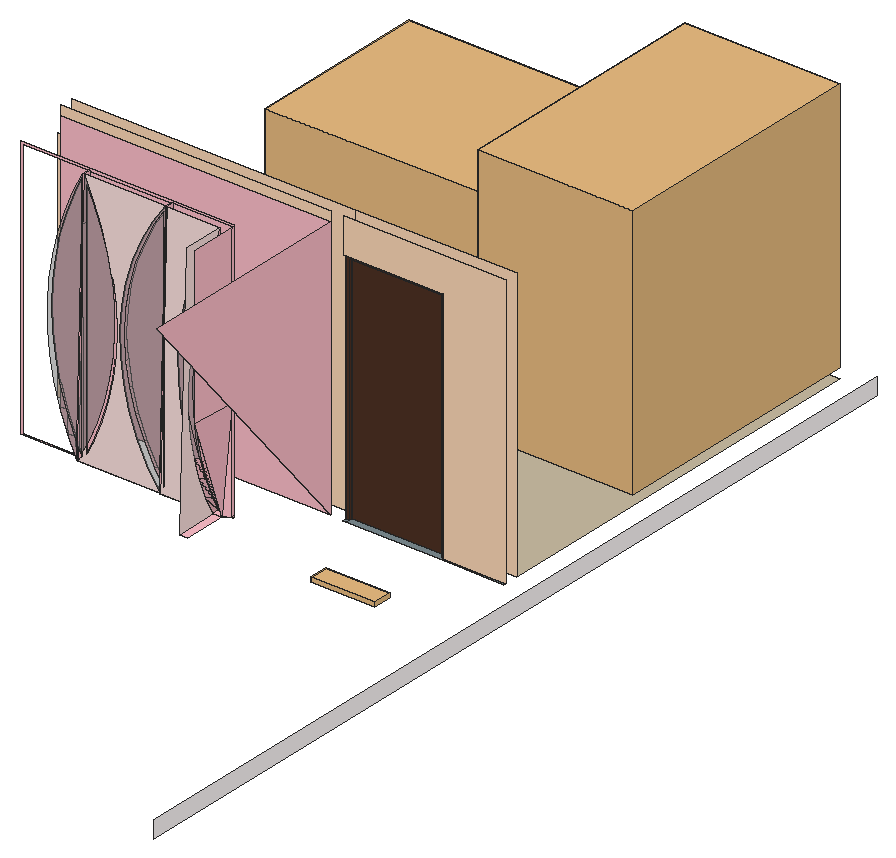
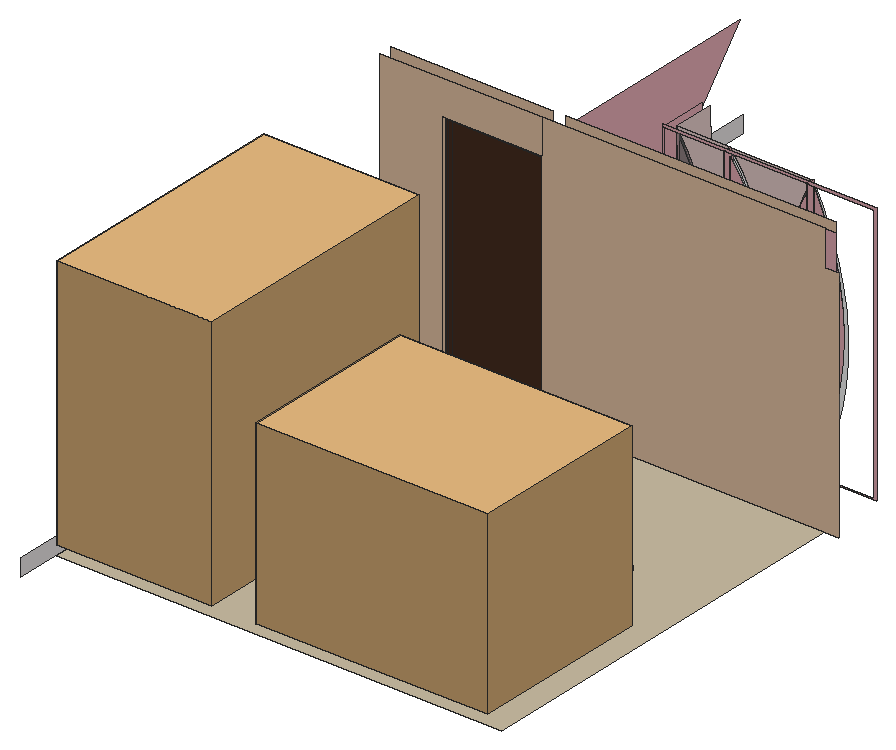
# SketchUp Ruby script. Lengths in inches.
U = 1.inch
M = Sketchup.active_model
def pt(a) = Geom::Point3d.new(a.map { |v| v * U })
def face(e, loops, mat)
  f = e.add_face(loops[0].map { |a| pt(a) })
  loops[1..].each { |l| e.add_face(l.map { |a| pt(a) }).erase! }
  f.material = f.back_material = mat if mat
  f
end
# faces: each face lists its corners as indices into pts; further lists are holes
def faces(e, pts, list, mat = nil) = list.each { |f| face(e, (f[0].is_a?(Array) ? f : [f]).map { |l| l.map { |i| pts[i] } }, mat) }
# xy, xz, yz: faces in a plane at the given z, y or x. An outline is a flat list of corners, or four numbers for a rectangle; further outlines are holes
def ring(l) = l.size == 4 ? [[l[0], l[1]], [l[2], l[1]], [l[2], l[3]], [l[0], l[3]]] : l.each_slice(2).to_a
def flat(e, list, mat, &to3) = list.each { |f| face(e, (f[0].is_a?(Array) ? f : [f]).map { |l| ring(l).map { |u, v| to3.(u, v) } }, mat) }
def xy(e, z, list, mat = nil) = flat(e, list, mat) { |x, y| [x, y, z] }
def xz(e, y, list, mat = nil) = flat(e, list, mat) { |x, z| [x, y, z] }
def yz(e, x, list, mat = nil) = flat(e, list, mat) { |y, z| [x, y, z] }
def lines(e, pts, list) = list.each { |a, b| e.add_line(pt(pts[a]), pt(pts[b])) }
# prism: a flat outline (further loops are holes) pulled along v
def prism(e, loops, v, mat = nil)
  f = face(e, loops, mat); d = Geom::Vector3d.new(v.map { |x| x * U })
  f.pushpull(f.normal.samedirection?(d) ? d.length : -d.length)
end
def box(e, o, s, mat = nil) = prism(e, [[o, [o[0] + s[0], o[1], o[2]], [o[0] + s[0], o[1] + s[1], o[2]], [o[0], o[1] + s[1], o[2]]]], [0, 0, s[2]], mat)
def at(x, y, z, deg = 0) = Geom::Transformation.translation(pt([x, y, z])) * Geom::Transformation.rotation(ORIGIN, Z_AXIS, deg.degrees)
def axes(o, x, y, z) = Geom::Transformation.new([*x, 0, *y, 0, *z, 0, *pt(o).to_a, 1])
def part(name) = M.definitions.add(name)
# library, detail: a bought-in or finely detailed component or shape, given as its bounding box
def library(name, o, s) = part(name).tap { |d| box(d.entities, o, s) }
def detail(e, o, s) = box(e.add_group.entities, o, s)
def put(e, d, t, mat = nil) = e.add_instance(d, t).tap { |i| i.material = mat if mat }
def group(e, t, mat = nil) = e.add_group.tap { |g| g.transformation = t; g.material = mat if mat }.entities
root = M.entities
M.materials.add("Polis06_194").color = [79, 50, 36]
M.materials.add("[0006_Pink]").color = [255, 192, 203]
M.materials.add("[0007_MistyRose]").color = [255, 228, 225]
M.materials.add("[0010_Snow]").color = [255, 250, 250]
M.materials.add("[0027_PeachPuff]").color = [255, 218, 185]
M.materials.add("[0093_AliceBlue]").color = [240, 248, 255]
M.materials.add("[Concrete Pavers Block Multi]").color = [124, 140, 145]
M.materials.add("[Concrete Tile]").color = [203, 190, 164]
M.materials.add("[Translucent Glass Gray]").color = [128, 128, 128]
M.materials["[Translucent Glass Gray]"].alpha = 0.5
c1 = library("Bedroom1",[0.98,0,0],[44.34,8.22,2])
c2 = library("Bed 003",[-38.05,-87.1,0],[75.86,87.1,55.12])
c3 = part("Flush door")
xy(c3.entities,0,[[0,0,4.72,1.18],[0,34.25,4.72,35.43]],"Polis06_194")
xy(c3.entities,85.26,[[0,1.18,4.72,34.25]],"Polis06_194")
xy(c3.entities,86.61,[[0,0,4.72,35.43]],"Polis06_194")
xz(c3.entities,0,[[0,0,4.72,86.61]],"Polis06_194")
xz(c3.entities,1.18,[[0,0,2.36,85.26],[2.36,0,4.72,85.26]],"Polis06_194")
xz(c3.entities,34.25,[[0,0,4.72,85.26]],"Polis06_194")
xz(c3.entities,35.43,[[0,0,4.72,86.61]],"Polis06_194")
yz(c3.entities,0,[[0,0,1.18,86.61],[34.25,0,35.43,86.61],[1.18,85.26,34.25,86.61]],"Polis06_194")
yz(c3.entities,2.36,[[1.18,0,34.25,0,34.25,85.21,1.18,85.26]],"Polis06_194")
yz(c3.entities,4.72,[[0,0,1.18,86.61],[34.25,0,35.43,86.61],[1.18,85.26,34.25,86.61]],"Polis06_194")
c4 = library("wardrobe\#1",[0.19,0,0],[43.3,8.22,2])
c5 = library("toilet 1",[0.13,0,0],[28.4,8.22,2])
xy(root,0,[[490.5625,345.21,492.04,347.21],[492.04,345.21,535.05,348.7],[535.05,345.21,562.5625,345.9375]],"[Concrete Pavers Block Multi]")
xy(root,0,[[492.04,348.7,533.35,350.1875],[490.5625,350.1875,534.83,351.9375],[364.5625,351.9375,562.5625,531.9375]],"[Concrete Tile]")
xy(root,0.5,[[453.1,301.65,453.1,320.15,429.42,320.15,429.42,320.52,456.54,320.52,456.54,301.65],[392.54,320.52,392.64,320.625,394.9375,321.02,394.9375,322.95,395.4375,323.46,431.8125,323.46,428.92,320.52],[429.42,320.52,432.3125,323.46,459.4375,323.46,459.4375,322.46,456.54,320.52],[392.64,320.625,393.03,321.02,394.9375,321.02],[393.03,321.02,394.9375,322.95,394.9375,321.02]],"[0006_Pink]")
xz(root,319.25,[[456,4.09,456.75,112.22]],"[0006_Pink]")
xz(root,320.15,[[454.84,4.76,454.84,69.55,453.28,7.4]],"[0006_Pink]")
xz(root,320.15,[[429.42,0.5,453.1,0.5,448.16,9.39,444.09,18.71,440.95,28.39,438.76,38.32,437.54,48.42,437.3,58.59,438.05,68.73,439.78,78.76,442.46,88.57,446.09,98.07,450.61,107.18,456,115.8125,432.3125,115.8125]],"[0007_MistyRose]")
xz(root,320.15,[[453.1,0.5,453.28,7.4,451.86,9.8,447.61,18.92,444.27,28.4,441.86,38.16,440.4,48.11,439.91,58.16,440.4,68.2,441.86,78.15,444.27,87.91,447.61,97.4,451.86,106.51,454.84,111.56,454.84,69.55,456,115.8125,450.61,107.18,446.09,98.07,442.46,88.57,439.78,78.76,438.05,68.73,437.3,58.59,437.54,48.42,438.76,38.32,440.95,28.39,444.09,18.71,448.16,9.39],[453.28,7.4,454.84,69.55,454.84,111.56,451.86,106.51,447.61,97.4,444.27,87.91,441.86,78.15,440.4,68.2,439.91,58.16,440.4,48.11,441.86,38.16,444.27,28.4,447.61,18.92,451.86,9.8]],"[Translucent Glass Gray]")
xz(root,320.52,[[392.54,0.5,394.09,3.36,392.6875,6.28],[394.45,2.62,394.45,4.02,394.09,3.36],[396.41,4.55,399.12,9.85,402.875,19.08,405.82,28.59,407.94,38.33,409.22,48.2,409.65,58.16,409.22,68.11,407.94,77.99,407.79,78.69,407.96,77.82,409,67.82,409.18,57.77,408.49,47.75,406.95,37.82,404.57,28.06,401.35,18.54,397.34,9.33,396.41,7.63]],"[0006_Pink]")
xz(root,320.52,[[392.54,0.5,428.92,0.5,423.43,9.21,418.9,18.46,415.38,28.14,412.92,38.14,411.53,48.34,411.24,58.64,412.05,68.9,413.94,79.02,416.91,88.89,420.91,98.375,425.89,107.39,431.8125,115.8125,395.4375,115.8125,399.78,106.75,403.33,97.35,406.07,87.68,407.79,78.69,407.94,77.99,409.22,68.11,409.65,58.16,409.22,48.2,407.94,38.33,405.82,28.59,402.875,19.08,399.12,9.85,396.41,4.55,396.41,7.63,394.45,4.02,394.45,2.62,394.09,3.36]],"[0007_MistyRose]")
xz(root,320.52,[[392.04,0.5,392.21,7.26,391.03,9.7,387.45,19,384.63,28.56,382.61,38.3125,381.39,48.2,380.98,58.16,381.39,68.11,382.61,78,384.63,87.76,387.45,97.31,391.03,106.61,394.45,113.69,394.45,96.52,394.9375,115.8125,390.36,106.91,386.53,97.67,383.46,88.14,381.1875,78.4,379.71,68.5,379.05,58.52,379.21,48.51,380.18,38.55,381.97,28.71,384.55,19.04,387.92,9.62],[428.92,0.5,429.06,6.18,426.85,9.51,422.13,18.55,418.41,28.05,415.71,37.89,414.09,47.97,413.54,58.16,414.09,68.35,415.71,78.42,418.41,88.26,422.13,97.76,426.85,106.81,430.96,112.99,430.96,81.8125,431.8125,115.8125,425.89,107.39,420.91,98.375,416.91,88.89,413.94,79.02,412.05,68.9,411.24,58.64,411.53,48.34,412.92,38.14,415.38,28.14,418.9,18.46,423.43,9.21],[394.09,3.36,394.45,4.02,394.45,76.61,392.6875,6.28],[394.45,4.02,396.41,7.63,396.41,111.77,399.12,106.46,402.875,97.23,405.82,87.72,407.79,78.69,406.07,87.68,403.33,97.35,399.78,106.75,395.4375,115.8125,394.45,76.61],[429.06,6.18,430.96,81.8125,430.96,112.99,426.85,106.81,422.13,97.76,418.41,88.26,415.71,78.42,414.09,68.35,413.54,58.16,414.09,47.97,415.71,37.89,418.41,28.05,422.13,18.55,426.85,9.51],
  [392.21,7.26,394.45,96.52,394.45,113.69,391.03,106.61,387.45,97.31,384.63,87.76,382.61,78,381.39,68.11,380.98,58.16,381.39,48.2,382.61,38.3125,384.63,28.56,387.45,19,391.03,9.7],[396.41,7.63,397.34,9.33,401.35,18.54,404.57,28.06,406.95,37.82,408.49,47.75,409.18,57.77,409,67.82,407.96,77.82,407.79,78.69,405.82,87.72,402.875,97.23,399.12,106.46,396.41,111.77]],"[Translucent Glass Gray]")
xz(root,320.9,[[396.41,4.55,399.12,9.85,402.875,19.08,405.82,28.59,407.94,38.33,409.22,48.2,409.65,58.16,409.22,68.11,407.94,77.99,405.82,87.72,402.875,97.23,399.12,106.46,396.41,111.77]],"[0006_Pink]")
xz(root,321.02,[[394.45,2.62,394.45,113.69,391.03,106.61,387.45,97.31,384.63,87.76,382.61,78,381.39,68.11,380.98,58.16,381.39,48.2,382.61,38.3125,384.63,28.56,387.45,19,391.03,9.7]],"[0006_Pink]")
xz(root,321.71,[[430.96,3.32,430.96,112.99,426.85,106.81,422.13,97.76,418.41,88.26,415.71,78.42,414.09,68.35,413.54,58.16,414.09,47.97,415.71,37.89,418.41,28.05,422.13,18.55,426.85,9.51]],"[0006_Pink]")
xz(root,323.46,[[[364.5625,0,459.4375,0,459.4375,0.5,432.3125,0.5,432.3125,115.8125,459.4375,115.8125,459.4375,116.8125,364.5625,116.8125],[395.4375,0.5,431.8125,115.8125],[365.5625,0.5,394.9375,115.8125]]],"[0006_Pink]")
xz(root,345.9375,[[364.5625,0,484.5625,116.8125]],"[0006_Pink]")
xz(root,345.9375,[[364.5625,0,484.5625,121.1875],[534.83,0,562.5625,0,562.5625,121.1875,490.5625,121.1875,490.5625,105.875,534.83,105.875]],"[0027_PeachPuff]")
xz(root,351.9375,[[358.5625,0,358.5625,105.53,364.5625,105.53,364.5625,121.1875,490.5625,121.1875,490.5625,0],[534.83,0,534.83,105.875,490.5625,105.875,490.5625,121.1875,562.5625,121.1875,562.5625,0]],"[0027_PeachPuff]")
yz(root,394.45,[[320.52,2.62,321.02,113.69]],"[0006_Pink]")
yz(root,394.9375,[[321.02,0.5,323.46,0.5,323.46,115.8125,320.52,115.8125]],"[0006_Pink]")
yz(root,396.41,[[320.52,4.55,320.9,111.77]],"[0006_Pink]")
yz(root,430.96,[[320.52,3.32,321.71,112.99]],"[0006_Pink]")
yz(root,431.8125,[[323.46,0.5,323.46,115.8125,320.52,115.8125]],"[0006_Pink]")
yz(root,456,[[319.25,4.09,316.19,9.78,312.27,18.98,309.18,28.5,306.96,38.25,305.625,48.16,305.18,58.16,305.625,68.15,306.96,78.0625,309.18,87.82,312.27,97.33,316.19,106.54,319.25,112.22]],"[Translucent Glass Gray]")
yz(root,456.75,[[319.25,4.09,319.25,112.22,316.19,106.54,312.27,97.33,309.18,87.82,306.96,78.0625,305.625,68.15,305.18,58.16,305.625,48.16,306.96,38.25,309.18,28.5,312.27,18.98,316.19,9.78]],"[0006_Pink]")
yz(root,459.4375,[[323.46,0,322.46,0.5,323.46,0.5],[322.46,0.5,322.46,45.68,323.46,45.625,323.46,0.5],[323.46,45.625,322.46,45.68,322.46,115.8125,323.46,115.8125],[322.46,45.68,322.46,115.8125,301.71,115.8125,301.71,46.85]],"[0006_Pink]")
yz(root,484.5625,[[345.9375,0,345.9375,116.8125,249.21,116.8125]],"[0006_Pink]")
yz(root,534.83,[[345.9375,0,351.9375,105.875]],"[0027_PeachPuff]")
yz(root,571.5625,[[138.9375,-7.5625,540.9375,0]],"[0010_Snow]")
p = [[459.4375,322.46,0.5],[459.4375,323.46,0],[456.54,320.52,0.5],[453.1,320.15,0.5],[453.1,301.65,0.5],[456,301.65,115.8125],
  [456,320.15,115.8125],[455.78,315.38,106.93],[455.54,311.42,97.65],[455.3,308.31,88.06],[455.06,306.07,78.22],[454.81,304.72,68.23],
  [454.55,304.27,58.16],[454.3,304.72,48.08],[454.05,306.07,38.09],[453.8,308.31,28.26],[453.56,311.42,18.66],[453.33,315.38,9.39],
  [459.4375,322.46,45.68],[459.4375,301.71,46.85],[456,319.25,4.09],[454.84,320.15,69.55],[453.28,320.15,7.4],[456,319.25,112.22],
  [432.3125,320.15,115.8125],[432.3125,323.46,115.8125],[429.42,320.52,0.5],[429.42,320.15,0.5],[387.92,320.52,9.62],[390.59,321.02,9.51],
  [392.04,320.52,0.5],[394.9375,321.02,0.5],[392.64,320.625,0.5],[394.9375,320.52,115.8125],[394.45,320.52,96.52],[392.21,320.52,7.26],
  [395.4375,323.46,0.5],[394.9375,322.95,0.5],[393.03,321.02,0.5],[392.54,320.52,0.5],[395.4375,323.46,115.8125],[395.4375,320.52,115.8125],
  [392.6875,320.52,6.28],[394.45,320.52,76.61],[428.92,320.52,0.5],[431.8125,323.46,0.5],[431.8125,320.52,115.8125],[430.96,320.52,81.8125],
  [429.06,320.52,6.18],[432.3125,323.46,0.5],[394.45,321.02,2.62],[391.03,321.02,9.7],[391.03,320.52,9.7],[394.09,320.52,3.36],
  [394.45,320.52,2.62],[426.85,320.52,9.51],[430.96,320.52,3.32],[430.96,321.71,3.32],[426.85,321.71,9.51],[456,316.19,9.78],
  [456.75,316.19,9.78],[456.75,319.25,4.09],[396.41,320.52,4.55],[399.12,320.52,9.85],[399.12,320.9,9.85],[396.41,320.9,4.55],
  [386.99,321.02,18.84],[422.13,320.52,18.55],[422.13,321.71,18.55],[384.55,320.52,19.04],[387.45,321.02,19],[387.45,320.52,19],
  [456,312.27,18.98],[456.75,312.27,18.98],[402.875,320.52,19.08],[402.875,320.9,19.08],[418.41,320.52,28.05],[418.41,321.71,28.05],
  [456,309.18,28.5],[456.75,309.18,28.5],[384.63,321.02,28.56],[384.63,320.52,28.56],[405.82,320.52,28.59],[405.82,320.9,28.59],
  [415.71,320.52,37.89],[415.71,321.71,37.89],[407.94,320.52,38.33],[407.94,320.9,38.33],[414.09,320.52,47.97],[414.09,321.71,47.97],
  [409.22,320.52,48.2],[409.22,320.9,48.2]]
faces(root,p,[[0,1,2],[18,19,2],[3,17,20],[6,21,22,3,23],[24,25,26,27],[28,29,30],[31,32,30,29],[32,31,33,34,35,30],
  [36,37,38,32,39,40],[41,40,39,42,43],[44,45,46,47,48],[49,26,25],[0,18,2],[50,51,52,35,42,53,54],[55,48,56,57,58],[59,20,17],
  [60,59,20,61],[62,63,64,65],[17,16,59],[29,28,66],[67,55,58,68],[69,66,28],[51,70,71,52],[72,59,16],
  [73,72,59,60],[63,74,75,64],[76,67,68,77],[16,15,72],[78,72,15],[79,78,72,73],[70,80,81,71],[74,82,83,75],
  [84,76,77,85],[82,86,87,83],[88,84,85,89],[86,90,91,87]],"[0006_Pink]")
faces(root,p,[[3,4,5,6,7,8,9,10,11,12,13,14,15,16,17]],"[0007_MistyRose]")
faces(root,p,[[20,23,3]],"[Translucent Glass Gray]")
detail(root,[493.45,416.65,4.375],[69.11,115.29,113.3])
put(root,c1,at(398.39,415.33,0))
put(root,c2,axes([427.22,526.02,0],[1.3566,0,0],[0,0.92,0],[0,0,1.449]),"[0093_AliceBlue]")
put(root,c3,axes([490.5625,350.1875,0],[0,-0.63,0],[1.24934,0,0],[0,0,1.22238]),"[0006_Pink]")
put(root,c4,at(499.46,479.17,0))
put(root,c5,at(509.07,304.53,0))
